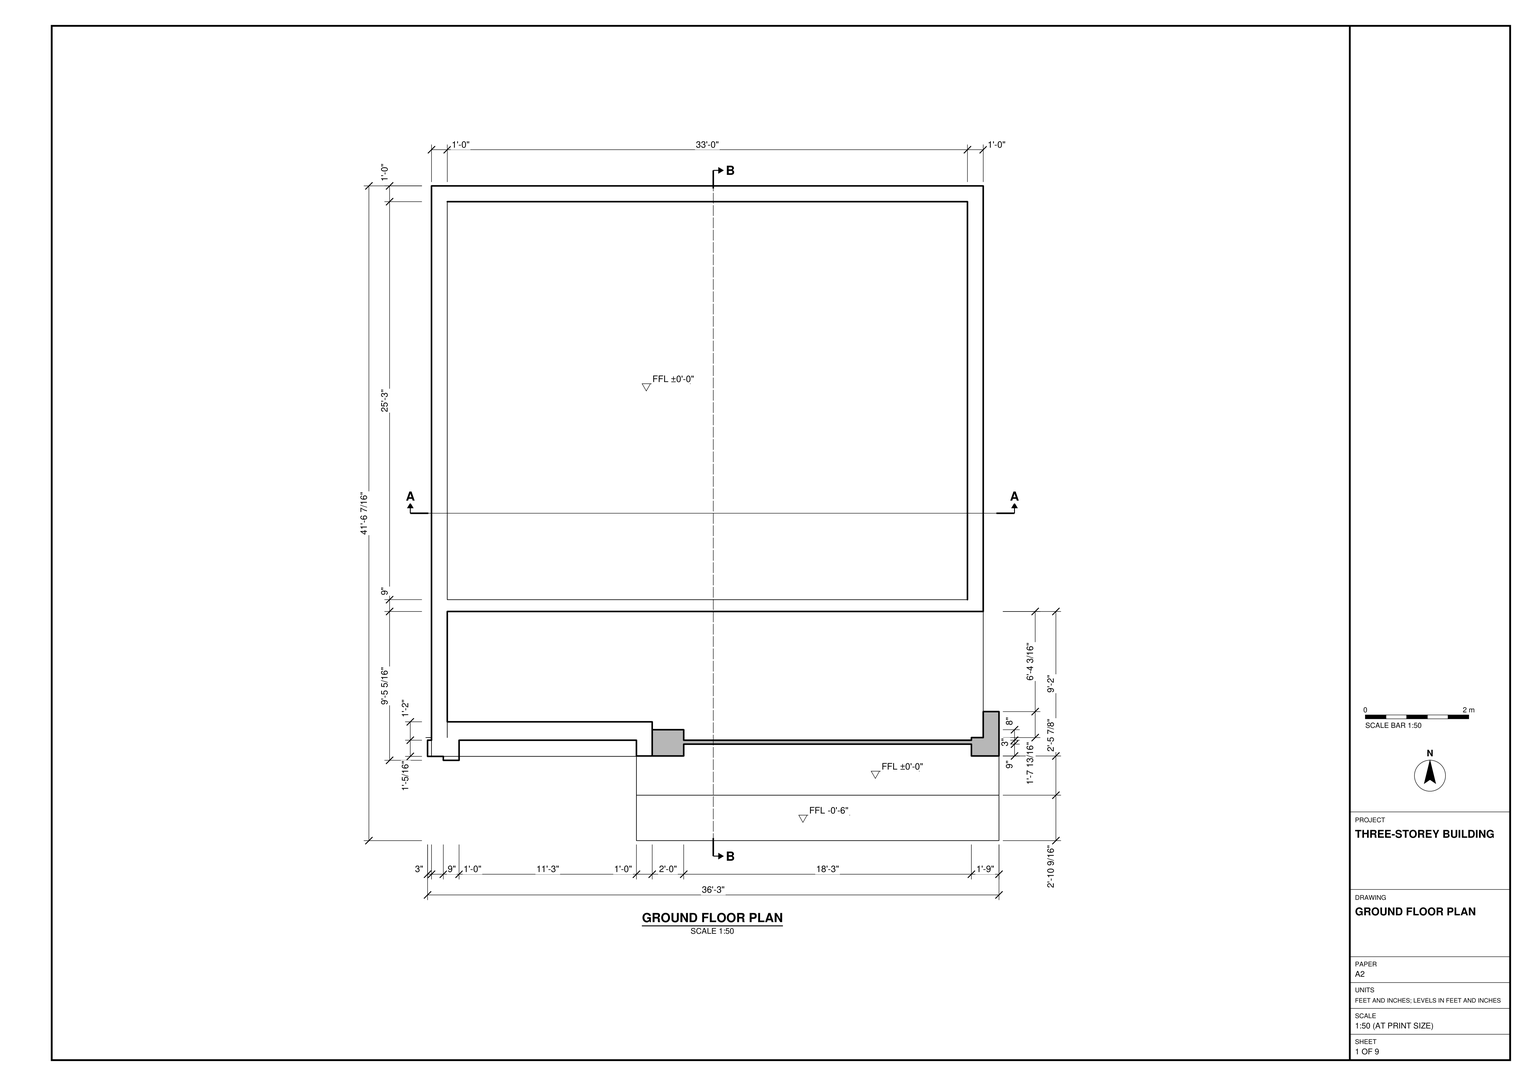
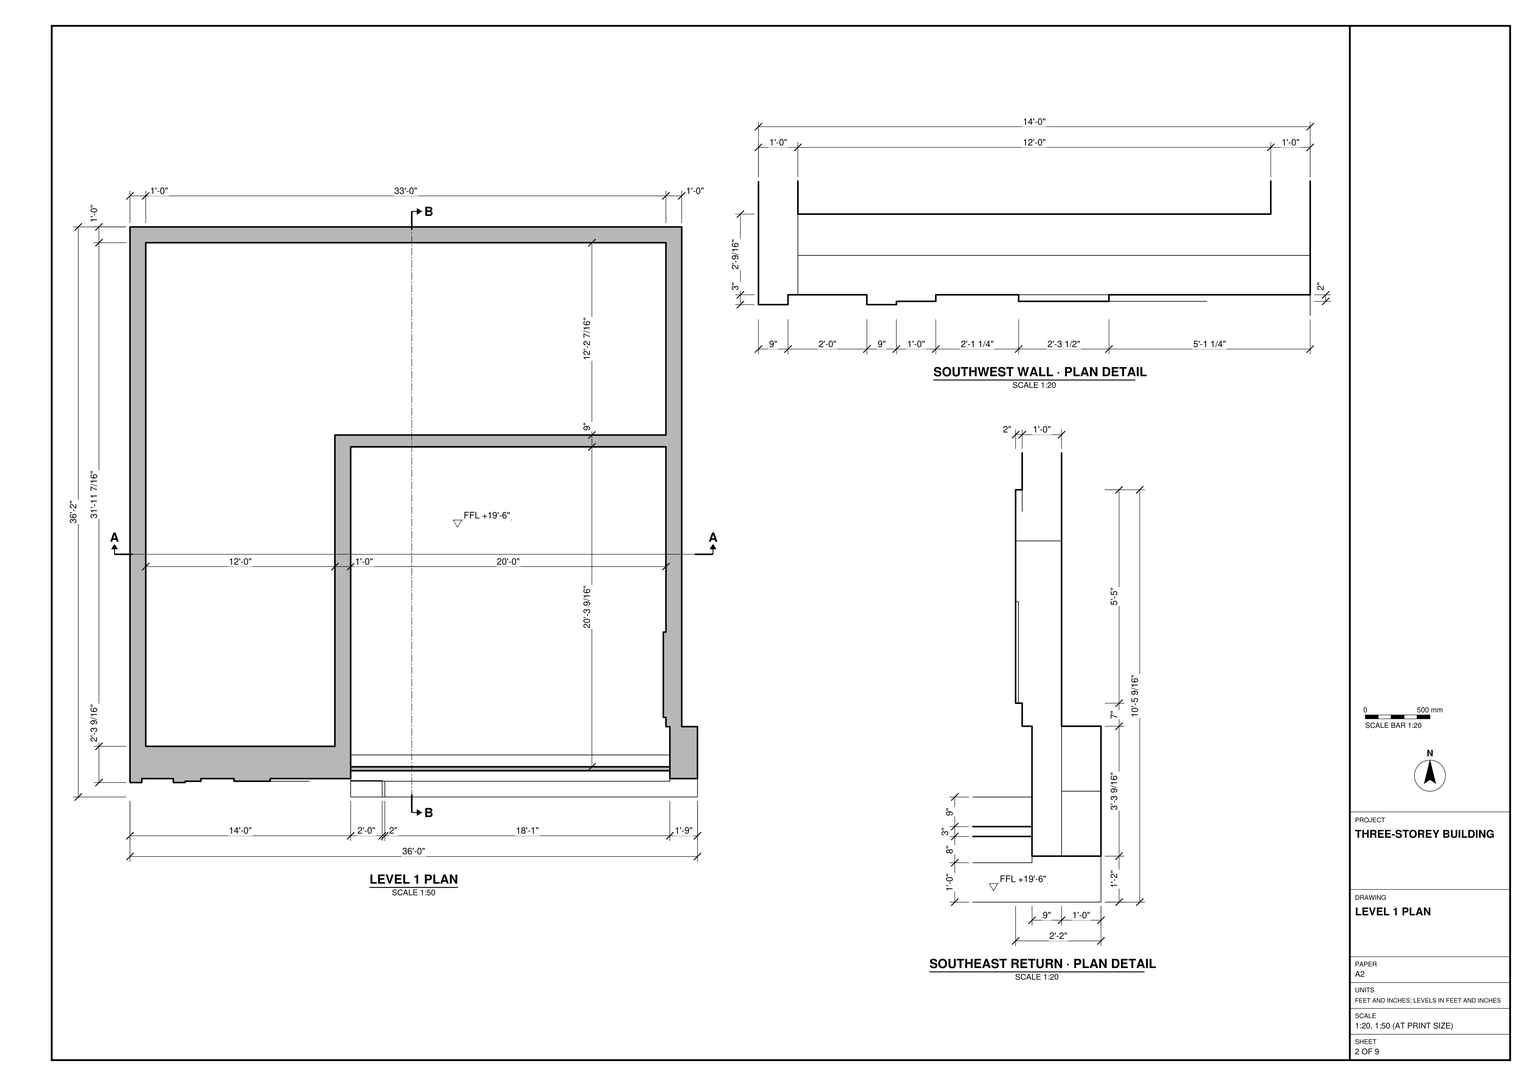
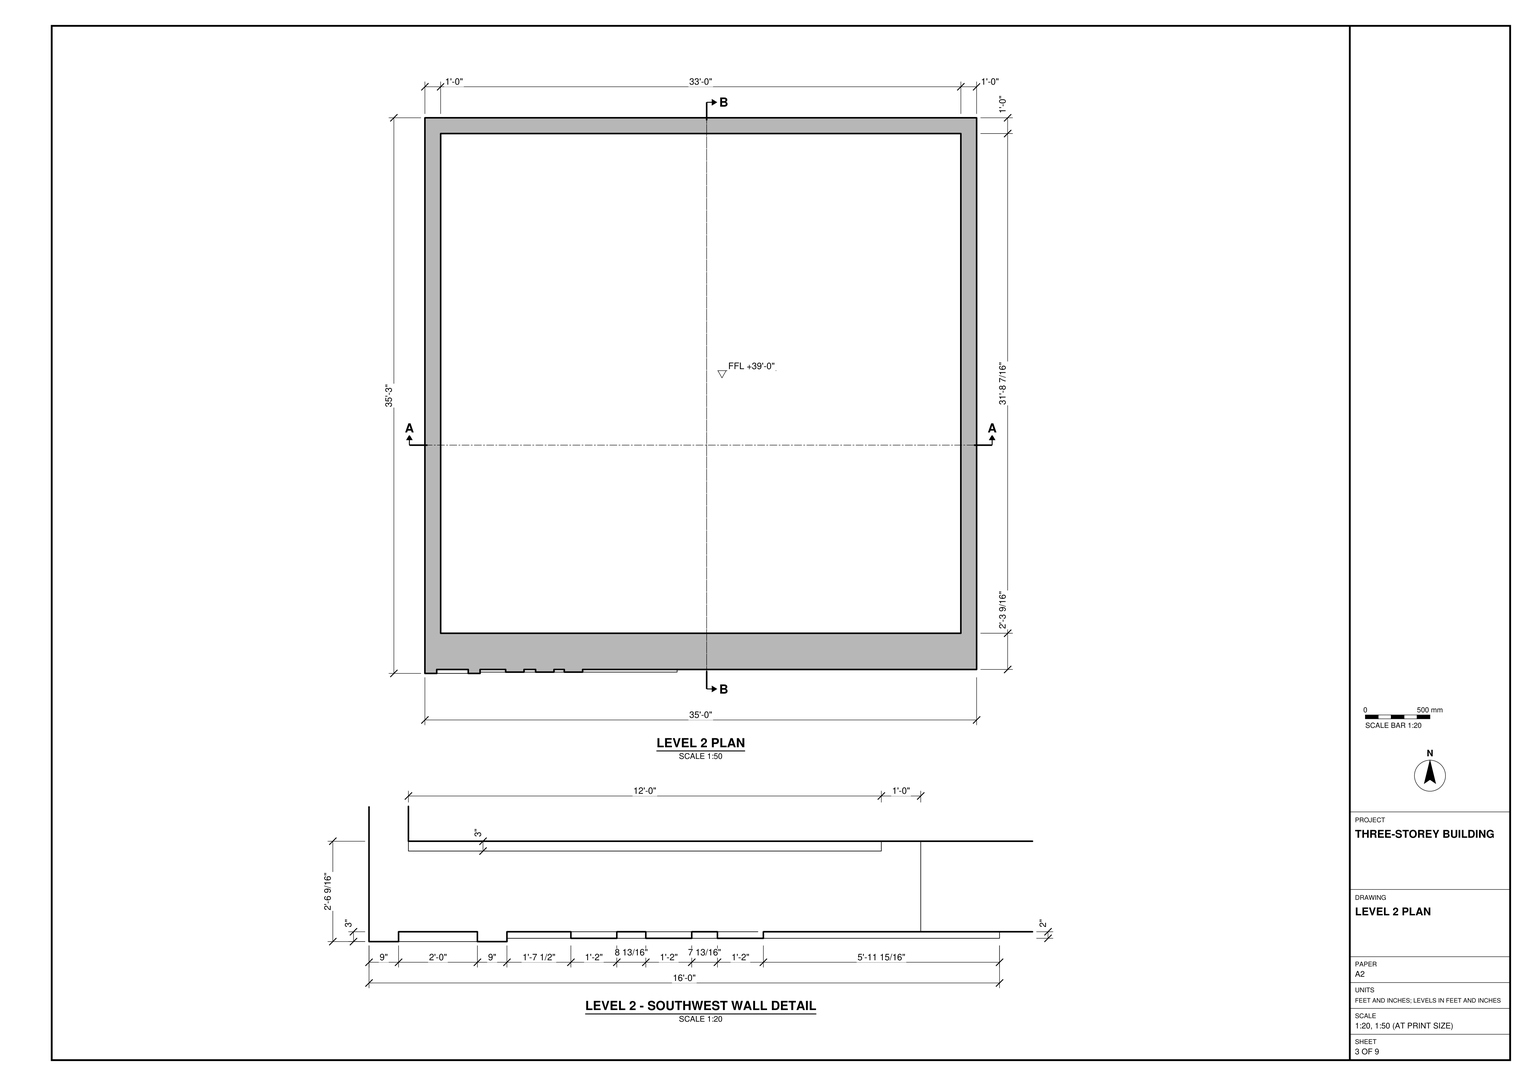
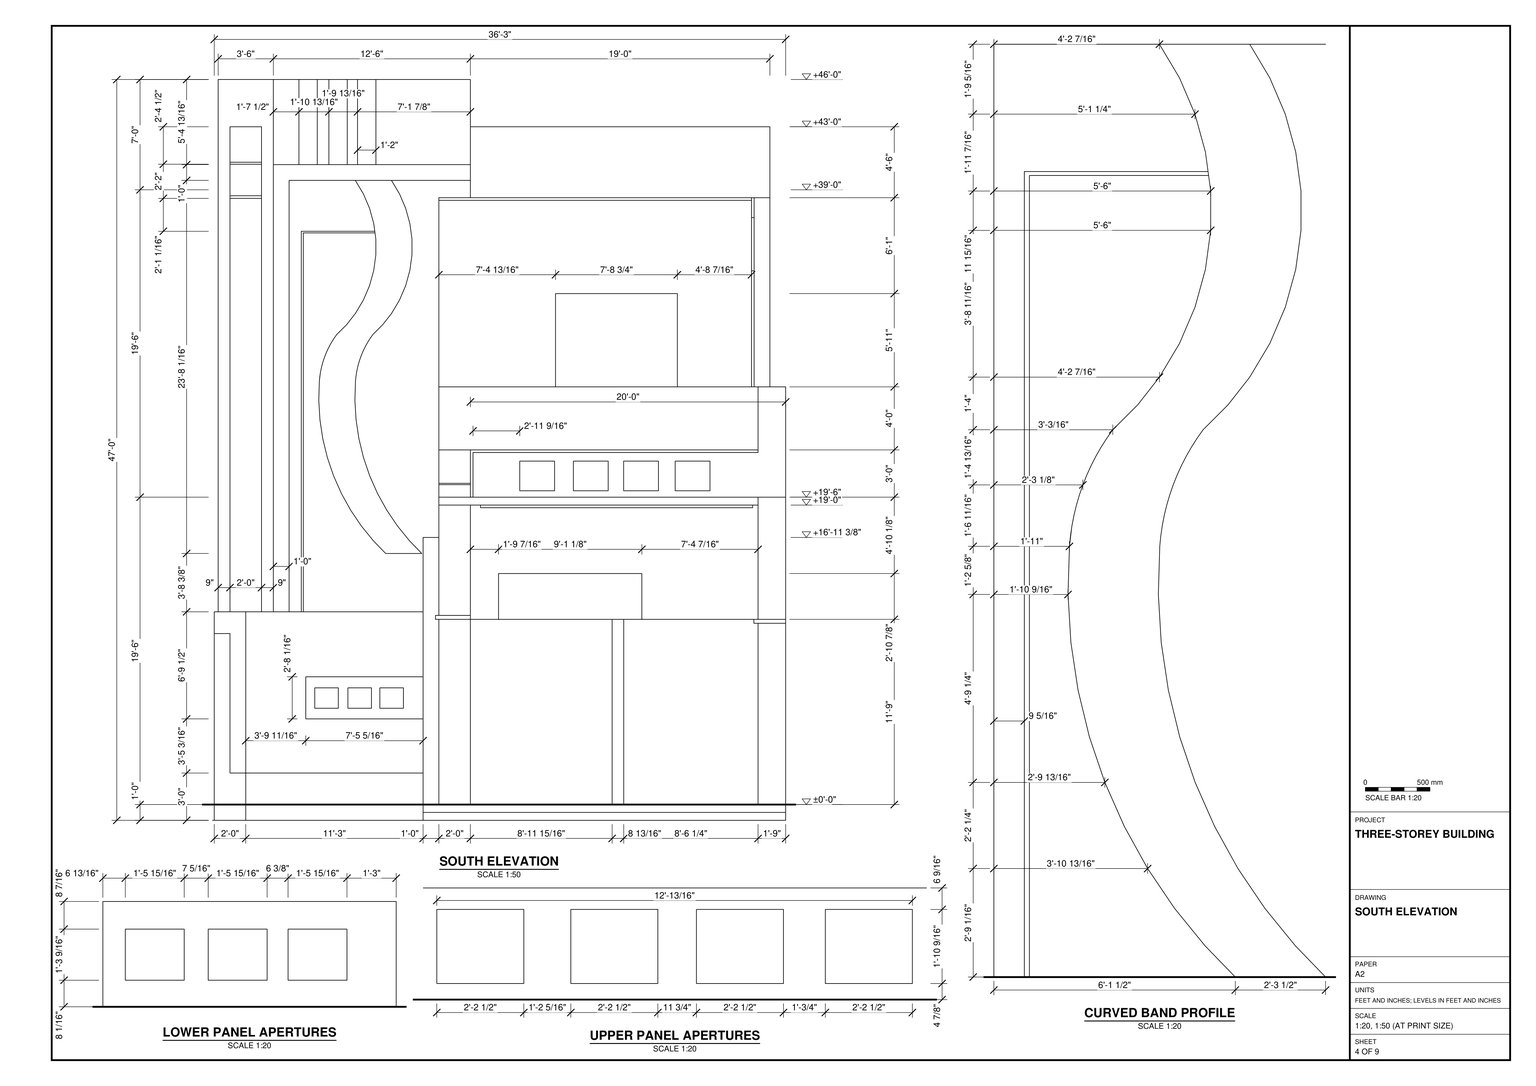
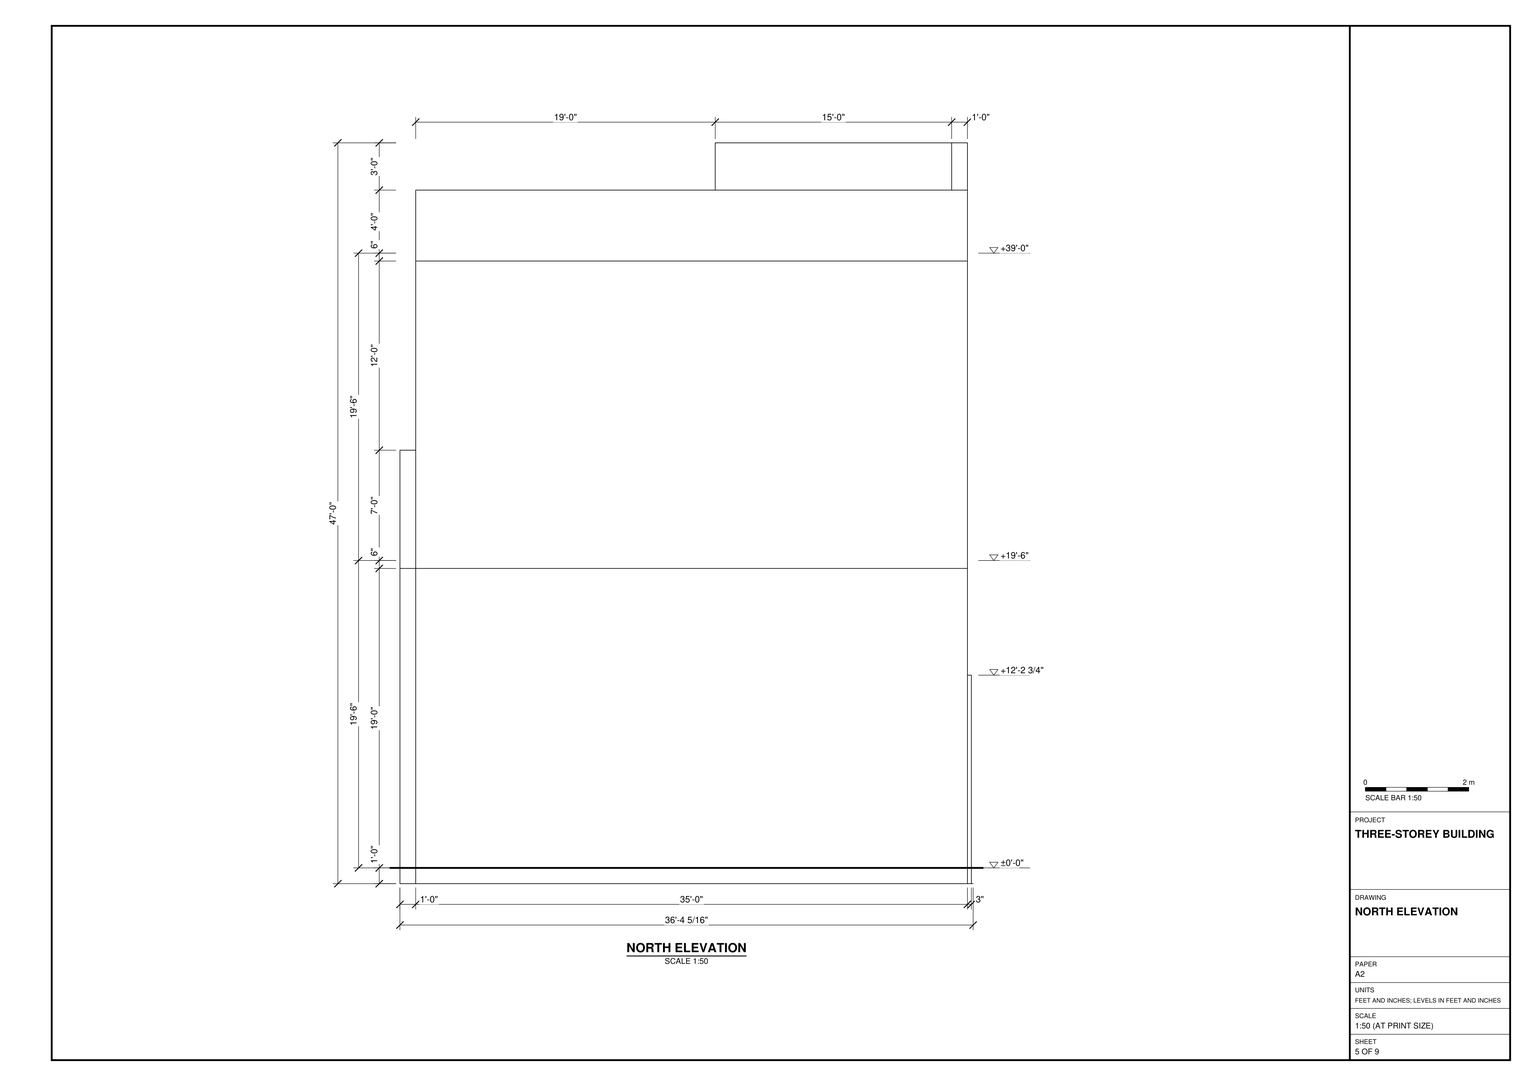
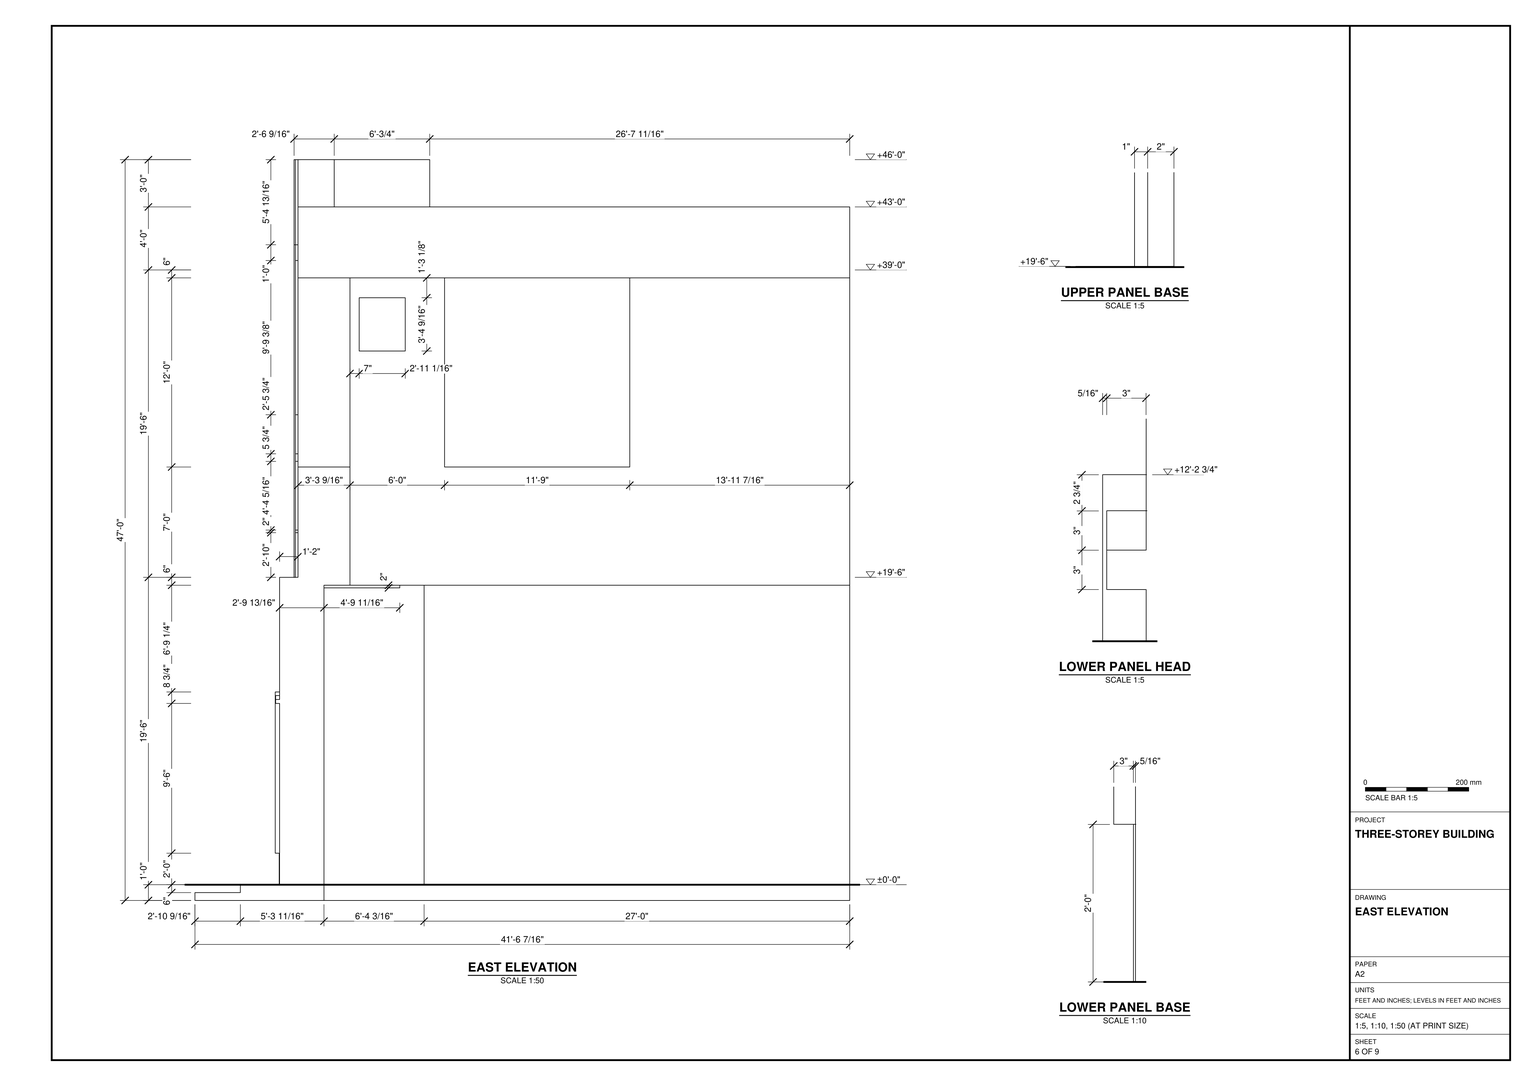
Build the three-storey shell in SketchUp from task_files/diagram_01.pdf. Work in feet and inches. Orient the south frontage along the x-axis. The overall model shall be 36'-3" wide, 41'-6 7/16" deep and 47'-0" high, including the projecting frontage and lower approach. Set the finished floor levels to ±0'-0", +19'-6" and +39'-0" relative to the ground floor.

Start with the rectangular ground-floor space. Use 1'-0" walls along its north, east and west sides and a 9" transverse wall separating it from the front zone. Model the stepped approach on the south side, including the lower strip in front of the eastern bay. At the middle level, use the Level 1 plan to locate the two walls that meet at the inset corner of the southeast bay. Follow the enlarged details for the offsets in the southwest wall face and the projecting southeast return. At the upper level, follow the rectangular perimeter and the thicker south edge. Use the sheets to resolve the openings, slab edges and roof profile rather than copying the same plan to every level.

Keep walls, slabs and roof elements in separate groups or components, do the same for each furniture or joinery piece shown, and use components for repeated parts. Any decor or loose items shown may be suitable library components. Save one SketchUp model as output_files/three_storey_building_with_its_stepped_south_frontage.skp.

# SketchUp Ruby script. Lengths in inches.
U = 1.inch
M = Sketchup.active_model
def pt(a) = Geom::Point3d.new(a.map { |v| v * U })
def face(e, loops, mat)
  f = e.add_face(loops[0].map { |a| pt(a) })
  loops[1..].each { |l| e.add_face(l.map { |a| pt(a) }).erase! }
  f.material = f.back_material = mat if mat
  f
end
# faces: each face lists its corners as indices into pts; further lists are holes
def faces(e, pts, list, mat = nil) = list.each { |f| face(e, (f[0].is_a?(Array) ? f : [f]).map { |l| l.map { |i| pts[i] } }, mat) }
# xy, xz, yz: faces in a plane at the given z, y or x. An outline is a flat list of corners, or four numbers for a rectangle; further outlines are holes
def ring(l) = l.size == 4 ? [[l[0], l[1]], [l[2], l[1]], [l[2], l[3]], [l[0], l[3]]] : l.each_slice(2).to_a
def flat(e, list, mat, &to3) = list.each { |f| face(e, (f[0].is_a?(Array) ? f : [f]).map { |l| ring(l).map { |u, v| to3.(u, v) } }, mat) }
def xy(e, z, list, mat = nil) = flat(e, list, mat) { |x, y| [x, y, z] }
def xz(e, y, list, mat = nil) = flat(e, list, mat) { |x, z| [x, y, z] }
def yz(e, x, list, mat = nil) = flat(e, list, mat) { |y, z| [x, y, z] }
def lines(e, pts, list) = list.each { |a, b| e.add_line(pt(pts[a]), pt(pts[b])) }
# prism: a flat outline (further loops are holes) pulled along v
def prism(e, loops, v, mat = nil)
  f = face(e, loops, mat); d = Geom::Vector3d.new(v.map { |x| x * U })
  f.pushpull(f.normal.samedirection?(d) ? d.length : -d.length)
end
def box(e, o, s, mat = nil) = prism(e, [[o, [o[0] + s[0], o[1], o[2]], [o[0] + s[0], o[1] + s[1], o[2]], [o[0], o[1] + s[1], o[2]]]], [0, 0, s[2]], mat)
def at(x, y, z, deg = 0) = Geom::Transformation.translation(pt([x, y, z])) * Geom::Transformation.rotation(ORIGIN, Z_AXIS, deg.degrees)
def axes(o, x, y, z) = Geom::Transformation.new([*x, 0, *y, 0, *z, 0, *pt(o).to_a, 1])
def part(name) = M.definitions.add(name)
# library, detail: a bought-in or finely detailed component or shape, given as its bounding box
def library(name, o, s) = part(name).tap { |d| box(d.entities, o, s) }
def detail(e, o, s) = box(e.add_group.entities, o, s)
def put(e, d, t, mat = nil) = e.add_instance(d, t).tap { |i| i.material = mat if mat }
def group(e, t, mat = nil) = e.add_group.tap { |g| g.transformation = t; g.material = mat if mat }.entities
root = M.entities
M.materials.add("[0005_LightPink]").color = [193, 138, 146]
M.materials.add("[0005_LightPink]1").color = [255, 182, 193]
M.materials.add("[0007_MistyRose]").color = [255, 228, 225]
M.materials.add("[0008_LavenderBlush]").color = [255, 240, 245]
M.materials.add("[0011_Seashell]").color = [255, 245, 238]
M.materials.add("[0012_Bisque]2").color = [255, 228, 196]
M.materials.add("[0013_LightCoral]").color = [255, 136, 136]
M.materials.add("[0013_LightCoral]1").color = [240, 128, 128]
M.materials.add("[0014_DarkSalmon]").color = [233, 150, 122]
M.materials.add("[0018_Brown]").color = [96, 24, 24]
M.materials.add("[0026_LightSalmon]").color = [255, 160, 122]
M.materials.add("[0111_SlateGray]").color = [112, 128, 144]
M.materials.add("[0119_RosyBrown]").color = [188, 143, 143]
M.materials.add("[0131_Silver]").color = [192, 192, 192]
M.materials.add("[0132_LightGray]").color = [169, 169, 169]
M.materials.add("[0136_Charcoal]").color = [35, 35, 35]
M.materials.add("[Brick Basket]").color = [230, 156, 152]
M.materials.add("[Brick Tumbled]").color = [135, 132, 132]
M.materials.add("[Carrera Marble]").color = [168, 168, 168]
M.materials.add("[Carrera Marble]1").color = [207, 207, 207]
M.materials.add("[Cladding Siding Tan]").color = [162, 126, 95]
M.materials.add("[Granite Dark Gray]").color = [69, 68, 68]
M.materials.add("[Stone Flagstone Ashlar]").color = [56, 37, 32]
M.materials.add("[Translucent Glass Gray]").color = [128, 128, 128]
M.materials["[Translucent Glass Gray]"].alpha = 0.5
M.materials.add("[Wood Cherry Original]").color = [152, 86, 42]
xy(root,0,[[159,0,159,76.4375,24,76.4375,24,64.125,3,64.125,3,498.4375,423,498.4375,423,98.221,435,98.221,435,0],[0,64.125,3,76.4375],[24,64.125,159,76.4375]])
xy(root,6,[[159,0,435,34.5625]],"[Granite Dark Gray]")
xy(root,12,[[171,64.4375,195,84.4375],[414,64.4375,435,78.4375],[195,73.4375,411,76.4375],[411,73.4375,414,76.4375],[423,78.4375,435,98.221],
  [15,183.4375,411,486.4375]])
xy(root,12,[[195,76.4375,414,76.4375,414,78.4375,423,78.4375,423,174.4375,15,174.4375,15,90.4375,171,90.4375,171,84.4375,195,84.4375]],"[Carrera Marble]")
xy(root,12,[[159,34.5625,435,34.5625,435,64.4375,414,64.4375,414,73.4375,195,73.4375,195,64.4375,159,64.4375]],"[Granite Dark Gray]")
xy(root,36,[[12,61.125,24,64.125]])
xy(root,36,[[24,64.125,159,76.4375]],"[Stone Flagstone Ashlar]")
xy(root,77.216,[[69.6875,70.4375,159,76.4375]],"[0111_SlateGray]")
xy(root,85.299,[[76.518,70.4375,94.455,72.4375],[101.768,70.4375,119.705,72.4375],[126.08,70.4375,144.018,72.4375]])
xy(root,100.862,[[76.518,70.4375,94.455,72.4375],[101.768,70.4375,119.705,72.4375],[126.08,70.4375,144.018,72.4375]])
xy(root,109.278,[[69.6875,70.4375,159,76.4375]],"[0111_SlateGray]")
xy(root,142.184,[[0,61.125,12,64.125]])
xy(root,150,[[410.8125,61.4375,410.8125,73.4375,414,73.4375,414,64.4375,435,64.4375,435,61.4375]])
xy(root,153,[[168.4375,61.4375,195,64.4375]])
xy(root,153,[[410.8125,61.4375,435,61.4375,435,64.4375,414,64.4375,414,76.4375,195,76.4375,195,73.4375,410.8125,73.4375]],"[0136_Charcoal]")
xy(root,156,[[168.4375,61.4375,195,61.4375,195,76.4375,171,76.4375,171,64.4375,168.4375,64.4375]],"[0013_LightCoral]")
xy(root,158.746,[[36,75.4375,45,76.4375]])
xy(root,158.746,[[0,61.125,24,61.125,24,76.4375,36,76.4375,36,78.4375,12,78.4375,12,75.4375,3,75.4375,3,76.4375,0,76.4375],[57,76.4375,159,78.4375]],"[0111_SlateGray]")
xy(root,203.132,[[130.514,76.4375,158.014,78.4375]],"[0026_LightSalmon]")
xy(root,215.357,[[171,78.4375,195,84.4375]])
xy(root,215.357,[[159,64.4375,171,78.4375]],"[0013_LightCoral]")
xy(root,238,[[237.548,105.396,235.982,105.433,234.479,105.874,233.141,106.689,232.06,107.822,231.309,109.197,230.94,110.719,230.976,112.285,231.417,113.788,232.232,115.125,233.366,116.207,234.74,116.958,236.262,117.327,237.828,117.29,239.331,116.849,240.669,116.034,241.75,114.901,242.501,113.527,242.87,112.004,242.834,110.439,242.393,108.936,241.578,107.598,240.444,106.517,239.07,105.766],[298.048,105.396,296.482,105.433,294.979,105.874,293.641,106.689,292.56,107.822,291.809,109.197,291.44,110.719,291.476,112.285,291.917,113.788,292.732,115.125,293.866,116.207,295.24,116.958,296.762,117.327,298.328,117.29,299.831,116.849,301.169,116.034,302.25,114.901,303.001,113.527,303.37,112.004,303.334,110.439,302.893,108.936,302.078,107.598,300.944,106.517,299.57,105.766],[341.735,105.396,340.169,105.433,338.666,105.874,337.329,106.689,336.248,107.822,335.497,109.197,335.127,110.719,335.164,112.285,335.605,113.788,336.42,115.125,337.553,116.207,338.928,116.958,340.45,117.327,342.016,117.29,343.519,116.849,344.856,116.034,345.9375,114.901,346.688,113.527,347.058,112.004,347.021,110.439,346.58,108.936,345.765,107.598,344.632,106.517,343.257,105.766],[386.048,105.396,384.482,105.433,382.979,105.874,381.641,106.689,380.56,107.822,379.809,109.197,379.44,110.719,379.476,112.285,379.917,113.788,380.732,115.125,381.866,116.207,383.24,116.958,384.762,117.327,386.328,117.29,387.831,116.849,389.169,116.034,390.25,114.901,391.001,113.527,391.37,112.004,391.334,110.439,390.893,108.936,390.078,107.598,388.944,106.517,387.57,105.766]])
xy(root,238,[[[202.693,81.739,409.88,155.927],[298.048,105.396,299.57,105.766,300.944,106.517,302.078,107.598,302.893,108.936,303.334,110.439,303.37,112.004,303.001,113.527,302.25,114.901,301.169,116.034,299.831,116.849,298.328,117.29,296.762,117.327,295.24,116.958,293.866,116.207,292.732,115.125,291.917,113.788,291.476,112.285,291.44,110.719,291.809,109.197,292.56,107.822,293.641,106.689,294.979,105.874,296.482,105.433],[386.048,105.396,387.57,105.766,388.944,106.517,390.078,107.598,390.893,108.936,391.334,110.439,391.37,112.004,391.001,113.527,390.25,114.901,389.169,116.034,387.831,116.849,386.328,117.29,384.762,117.327,383.24,116.958,381.866,116.207,380.732,115.125,379.917,113.788,379.476,112.285,379.44,110.719,379.809,109.197,380.56,107.822,381.641,106.689,382.979,105.874,384.482,105.433],[341.735,105.396,343.257,105.766,344.632,106.517,345.765,107.598,346.58,108.936,347.021,110.439,347.058,112.004,346.688,113.527,345.9375,114.901,344.856,116.034,343.519,116.849,342.016,117.29,340.45,117.327,338.928,116.958,337.553,116.207,336.42,115.125,335.605,113.788,335.164,112.285,335.127,110.719,335.497,109.197,336.248,107.822,337.329,106.689,338.666,105.874,340.169,105.433],[237.548,105.396,239.07,105.766,240.444,106.517,241.578,107.598,242.393,108.936,242.834,110.439,242.87,112.004,242.501,113.527,241.75,114.901,240.669,116.034,239.331,116.849,237.828,117.29,236.262,117.327,234.74,116.958,233.366,116.207,232.232,115.125,231.417,113.788,230.976,112.285,230.94,110.719,231.309,109.197,232.06,107.822,233.141,106.689,234.479,105.874,235.982,105.433]]],"[Wood Cherry Original]")
xy(root,240,[[321.222,67.739,319.656,67.776,318.153,68.217,316.816,69.032,315.734,70.165,314.983,71.54,314.614,73.062,314.651,74.628,315.092,76.131,315.906,77.468,317.04,78.549,318.414,79.3,319.936,79.67,321.502,79.633,323.005,79.192,324.343,78.377,325.424,77.244,326.175,75.869,326.545,74.347,326.508,72.782,326.067,71.279,325.252,69.941,324.119,68.86,322.744,68.109],[423,98.221,435,118.005]])
xy(root,240,[[[171,64.4375,171,76.4375,195,76.4375,195,78.4375,171,78.4375,171,90.4375,15,90.4375,15,174.4375,423,174.4375,423,78.4375,414,78.4375,414,64.4375],[202.693,81.739,409.88,155.927],[321.222,67.739,322.744,68.109,324.119,68.86,325.252,69.941,326.067,71.279,326.508,72.782,326.545,74.347,326.175,75.869,325.424,77.244,324.343,78.377,323.005,79.192,321.502,79.633,319.936,79.67,318.414,79.3,317.04,78.549,315.906,77.468,315.092,76.131,314.651,74.628,314.614,73.062,314.983,71.54,315.734,70.165,316.816,69.032,318.153,68.217,319.656,67.776]]],"[0007_MistyRose]")
xy(root,246,[[195,76.4375,197,78.4375],[171,77,195,78.4375],[15,103.005,159,103.005,159,340.005,411,340.005,411,486.4375,15,486.4375]])
xy(root,246,[[171,64.4375,195,77],[195,64.4375,197,76.4375],[197,64.4375,435,78.4375]],"[0111_SlateGray]")
xy(root,246,[[171,96.4375,414,96.4375,414,118.005,411,118.005,411,125.019,409,125.019,409,190.005,411,190.005,411,331.005,171,331.005]],"[Carrera Marble]")
xy(root,250.897,[[232.592,78.4375,259.092,81.4375],[273.405,78.4375,299.905,81.4375],[311.655,78.4375,338.155,81.4375],[350.905,78.4375,377.405,81.4375]],"[0111_SlateGray]")
xy(root,255.554,[[171,76.4375,195,77]])
xy(root,256.554,[[171,76.4375,195,77]])
xy(root,273.46,[[232.592,78.4375,259.092,81.4375],[273.405,78.4375,299.905,81.4375],[311.655,78.4375,338.155,81.4375],[350.905,78.4375,377.405,81.4375]])
xy(root,280,[[197,76.4375,414,78.4375]],"[0111_SlateGray]")
xy(root,282,[[171,84.4375,414,96.4375]])
xy(root,282,[[195,76.4375,414,76.4375,414,84.4375,171,84.4375,171,77,195,77]],"[0111_SlateGray]")
xy(root,330,[[411,190.005,423,331.005]],"[0005_LightPink]1")
xy(root,330,[[414,78.4375,435,118.005],[171,84.4375,414,87.4375]],"[0013_LightCoral]")
xy(root,418.301,[[409,125.019,423,160.081]],"[0005_LightPink]1")
xy(root,472,[[171,185.005,409,190.005]],"[Wood Cherry Original]")
xy(root,473.496,[[12,75.4375,36,78.4375]])
xy(root,474,[[218.054,111.37,216.501,111.574,215.054,112.173,213.812,113.127,212.858,114.37,212.259,115.817,212.054,117.37,212.259,118.923,212.858,120.37,213.812,121.612,215.054,122.566,216.501,123.165,218.054,123.37,219.607,123.165,221.054,122.566,222.297,121.612,223.25,120.37,223.85,118.923,224.054,117.37,223.85,115.817,223.25,114.37,222.297,113.127,221.054,112.173,219.607,111.574],[319.992,111.37,318.439,111.574,316.992,112.173,315.749,113.127,314.796,114.37,314.196,115.817,313.992,117.37,314.196,118.923,314.796,120.37,315.749,121.612,316.992,122.566,318.439,123.165,319.992,123.37,321.545,123.165,322.992,122.566,324.234,121.612,325.188,120.37,325.787,118.923,325.992,117.37,325.787,115.817,325.188,114.37,324.234,113.127,322.992,112.173,321.545,111.574],[219.3,215.462,217.747,215.666,216.3,216.266,215.058,217.219,214.104,218.462,213.505,219.909,213.3,221.462,213.505,223.015,214.104,224.462,215.058,225.705,216.3,226.658,217.747,227.258,219.3,227.462,220.853,227.258,222.3,226.658,223.543,225.705,224.497,224.462,225.096,223.015,225.3,221.462,225.096,219.909,224.497,218.462,223.543,217.219,222.3,216.266,220.853,215.666],[290.738,215.462,289.185,215.666,287.738,216.266,286.495,217.219,285.542,218.462,284.942,219.909,284.738,221.462,284.942,223.015,285.542,224.462,286.495,225.705,287.738,226.658,289.185,227.258,290.738,227.462,292.291,227.258,293.738,226.658,294.981,225.705,295.934,224.462,296.533,223.015,296.738,221.462,296.533,219.909,295.934,218.462,294.981,217.219,293.738,216.266,292.291,215.666],[372.738,215.462,371.185,215.666,369.738,216.266,368.495,217.219,367.542,218.462,366.942,219.909,366.738,221.462,366.942,223.015,367.542,224.462,368.495,225.705,369.738,226.658,371.185,227.258,372.738,227.462,374.291,227.258,375.738,226.658,376.981,225.705,377.934,224.462,378.533,223.015,378.738,221.462,378.533,219.909,377.934,218.462,376.981,217.219,375.738,216.266,374.291,215.666]])
xy(root,474,[[[171,78.4375,171,185.005,409,185.005,409,160.081,411,160.081,411,118.005,423,118.005,423,78.4375],[218.054,111.37,219.607,111.574,221.054,112.173,222.297,113.127,223.25,114.37,223.85,115.817,224.054,117.37,223.85,118.923,223.25,120.37,222.297,121.612,221.054,122.566,219.607,123.165,218.054,123.37,216.501,123.165,215.054,122.566,213.812,121.612,212.858,120.37,212.259,118.923,212.054,117.37,212.259,115.817,212.858,114.37,213.812,113.127,215.054,112.173,216.501,111.574],[319.992,111.37,321.545,111.574,322.992,112.173,324.234,113.127,325.188,114.37,325.787,115.817,325.992,117.37,325.787,118.923,325.188,120.37,324.234,121.612,322.992,122.566,321.545,123.165,319.992,123.37,318.439,123.165,316.992,122.566,315.749,121.612,314.796,120.37,314.196,118.923,313.992,117.37,314.196,115.817,314.796,114.37,315.749,113.127,316.992,112.173,318.439,111.574]],[[171,190.005,423,331.005],[290.738,215.462,292.291,215.666,293.738,216.266,294.981,217.219,295.934,218.462,296.533,219.909,296.738,221.462,296.533,223.015,295.934,224.462,294.981,225.705,293.738,226.658,292.291,227.258,290.738,227.462,289.185,227.258,287.738,226.658,286.495,225.705,285.542,224.462,284.942,223.015,284.738,221.462,284.942,219.909,285.542,218.462,286.495,217.219,287.738,216.266,289.185,215.666],[372.738,215.462,374.291,215.666,375.738,216.266,376.981,217.219,377.934,218.462,378.533,219.909,378.738,221.462,378.533,223.015,377.934,224.462,376.981,225.705,375.738,226.658,374.291,227.258,372.738,227.462,371.185,227.258,369.738,226.658,368.495,225.705,367.542,224.462,366.942,223.015,366.738,221.462,366.942,219.909,367.542,218.462,368.495,217.219,369.738,216.266,371.185,215.666],[219.3,215.462,220.853,215.666,222.3,216.266,223.543,217.219,224.497,218.462,225.096,219.909,225.3,221.462,225.096,223.015,224.497,224.462,223.543,225.705,222.3,226.658,220.853,227.258,219.3,227.462,217.747,227.258,216.3,226.658,215.058,225.705,214.104,224.462,213.505,223.015,213.3,221.462,213.505,219.909,214.104,218.462,215.058,217.219,216.3,216.266,217.747,215.666]]],"[Wood Cherry Original]")
xy(root,475.496,[[12,75.4375,36,78.4375]])
xy(root,480,[[15,106.005,411,486.4375]])
xy(root,487.191,[[57,76.4375,107.413,78.4375],[134.913,76.4375,195,78.4375]])
xy(root,499.191,[[45,76.4375,64.474,78.4375],[78.457,76.4375,87.286,78.4375],[101.27,76.4375,109.099,78.4375],[123.082,76.4375,195,78.4375]])
xy(root,499.496,[[12,75.4375,36,78.4375]])
xy(root,500.996,[[12,75.4375,36,78.4375]])
xy(root,528,[[12,75.4375,36,78.4375],[195,78.4375,423,78.4375,423,498.4375,3,498.4375,3,178.725,15,178.725,15,486.4375,411,486.4375,411,106.005,195,106.005]])
xy(root,564,[[3,75.4375,45,75.4375,45,78.4375,64.474,78.4375,64.474,76.4375,78.457,76.4375,78.457,78.4375,87.286,78.4375,87.286,76.4375,101.27,76.4375,101.27,78.4375,109.099,78.4375,109.099,76.4375,123.082,76.4375,123.082,78.4375,195,78.4375,195,106.005,15,106.005,15,178.725,3,178.725]])
xz(root,0,[[159,0,435,6]],"[Granite Dark Gray]")
xz(root,34.5625,[[159,6,435,12]],"[Granite Dark Gray]")
xz(root,61.125,[[12,36,24,36,24,158.746,0,158.746,0,142.184,12,142.184]],"[0111_SlateGray]")
xz(root,61.4375,[[168.4375,153,195,156]])
xz(root,61.4375,[[410.8125,150,435,153]],"[0013_LightCoral]")
xz(root,64.125,[[0,0,24,0,24,36,12,36,12,142.184,0,142.184],[24,0,159,36]],"[Stone Flagstone Ashlar]")
xz(root,64.4375,[[168.4375,153,171,156]])
xz(root,64.4375,[[159,12,171,12,171,153,168.4375,153,168.4375,156,171,156,171,215.357,159,215.357],[171,12,195,153],[414,12,435,150],[414,153,435,246]],"[0013_LightCoral]")
xz(root,64.4375,[[171,240,414,246]],"[0111_SlateGray]")
xz(root,70.4375,[[[69.6875,77.216,159,109.278],[76.518,85.299,94.455,100.862],[101.768,85.299,119.705,100.862],[126.08,85.299,144.018,100.862]]],"[0111_SlateGray]")
xz(root,72.4375,[[76.518,85.299,94.455,100.862],[101.768,85.299,119.705,100.862],[126.08,85.299,144.018,100.862]])
xz(root,73.4375,[[302.906,12,311.725,153]],"[0136_Charcoal]")
xz(root,73.4375,[[195,12,302.906,153],[311.725,12,414,12,414,150,410.8125,150,410.8125,153,311.725,153]],"[Cladding Siding Tan]")
xz(root,75.4375,[[12,473.496,36,475.496],[12,499.496,36,500.996]],"[0012_Bisque]2")
xz(root,75.4375,[[3,158.746,12,158.746,12,528,36,528,36,158.746,45,158.746,45,564,3,564]],"[Brick Basket]")
xz(root,76.4375,[[0,0,3,158.746],[24,0,159,36]])
xz(root,76.4375,[[45,158.746,57,158.746,57,487.191,195,487.191,195,499.191,45,499.191]],"[0005_LightPink]")
xz(root,76.4375,[[64.474,499.191,78.457,564],[87.286,499.191,101.27,564],[109.099,499.191,123.082,564]],"[0011_Seashell]")
xz(root,76.4375,[[171,156,195,240]],"[0013_LightCoral]")
xz(root,76.4375,[[130.514,203.132,158.014,203.132,148.792,212.666,139.533,224.026,131.322,236.166,124.225,248.988,118.298,262.391,113.588,276.269,110.132,290.51,107.958,305.004,107.084,319.633,107.515,334.281,107.826,337.465,108.202,340.047,108.287,340.631,108.895,343.771,109.651,346.879,110.551,349.949,111.595,352.973,112.779,355.944,114.102,358.857,115.559,361.704,117.149,364.48,118.868,367.178,120.711,369.792,128.295,377.376,134.913,385.816,141.044,396.099,145.741,407.111,148.921,418.653,150.525,430.517,150.525,442.489,148.921,454.353,145.741,465.895,141.044,476.907,134.913,487.191,107.413,487.191,113.544,476.907,118.241,465.895,121.421,454.353,123.025,442.489,123.025,430.517,121.421,418.653,118.241,407.111,113.544,396.099,107.413,385.816,100.795,377.376,93.211,369.792,91.368,367.178,89.649,364.48,88.059,361.704,86.602,358.857,85.279,355.944,84.095,352.973,83.051,349.949,82.151,346.879,81.395,343.771,80.787,340.631,80.702,340.047,80.015,334.281,79.584,319.633,80.458,305.004,82.632,290.51,86.088,276.269,90.798,262.391,96.725,248.988,103.822,236.166,112.033,224.026,121.292,212.666]],"[0026_LightSalmon]")
xz(root,76.4375,[[195,246,197,246,197,280,414,280,414,282,195,282],[171,255.554,195,256.554]],"[0111_SlateGray]")
xz(root,76.4375,[[24,36,159,36,159,77.216,69.6875,77.216,69.6875,109.278,159,109.278,159,158.746,24,158.746]],"[0132_LightGray]")
xz(root,76.4375,[[195,12,414,153]],"[Cladding Siding Tan]")
xz(root,77,[[171,246,195,255.554],[171,256.554,195,282]],"[0111_SlateGray]")
xz(root,78.4375,[[414,12,423,240],[66.285,158.746,67.823,158.746,67.823,447.223,122.385,447.223,122.223,448.421,66.285,448.421],[171,215.357,195,240],[80.015,334.281,80.702,340.047,80.326,337.465]])
xz(root,78.4375,[[57,158.746,66.285,158.746,66.285,448.421,122.223,448.421,121.421,454.353,118.241,465.895,113.544,476.907,107.413,487.191,57,487.191]],"[0005_LightPink]")
xz(root,78.4375,[[[197,246,435,246,435,330,414,330,414,280,197,280],[350.905,250.897,377.405,273.46],[311.655,250.897,338.155,273.46],[273.405,250.897,299.905,273.46],[232.592,250.897,259.092,273.46]]],"[0013_LightCoral]")
xz(root,78.4375,[[67.823,158.746,159,158.746,159,215.357,171,215.357,171,474,195,474,195,487.191,134.913,487.191,141.044,476.907,145.741,465.895,148.921,454.353,150.525,442.489,150.525,430.517,148.921,418.653,145.741,407.111,141.044,396.099,134.913,385.816,128.295,377.376,120.711,369.792,118.868,367.178,117.149,364.48,115.559,361.704,114.102,358.857,112.779,355.944,111.595,352.973,110.551,349.949,109.651,346.879,108.895,343.771,108.287,340.631,108.202,340.047,107.826,337.465,107.515,334.281,107.084,319.633,107.958,305.004,110.132,290.51,113.588,276.269,118.298,262.391,124.225,248.988,131.322,236.166,139.533,224.026,148.792,212.666,158.014,203.132,130.514,203.132,121.292,212.666,112.033,224.026,103.822,236.166,96.725,248.988,90.798,262.391,86.088,276.269,82.632,290.51,80.458,305.004,79.584,319.633,80.015,334.281,80.326,337.465,80.702,340.047,80.787,340.631,81.395,343.771,82.151,346.879,83.051,349.949,84.095,352.973,85.279,355.944,86.602,358.857,88.059,361.704,89.649,364.48,91.368,367.178,93.211,369.792,100.795,377.376,107.413,385.816,113.544,396.099,118.241,407.111,121.421,418.653,123.025,430.517,123.025,442.489,122.385,447.223,67.823,447.223]],"[0119_RosyBrown]")
xz(root,78.4375,[[45,499.191,64.474,564],[78.457,499.191,87.286,564],[101.27,499.191,109.099,564],[123.082,499.191,195,564]],"[Brick Basket]")
xz(root,78.4375,[[195,474,423,528]],"[Brick Tumbled]")
xz(root,78.4375,[[12,158.746,36,473.496],[12,475.496,36,499.496],[12,500.996,36,528]],"[Translucent Glass Gray]")
xz(root,81.4375,[[232.592,250.897,259.092,273.46],[273.405,250.897,299.905,273.46],[311.655,250.897,338.155,273.46],[350.905,250.897,377.405,273.46]],"[0111_SlateGray]")
xz(root,81.739,[[202.693,238,409.88,240]],"[Wood Cherry Original]")
xz(root,84.4375,[[171,12,195,215.357]],"[0007_MistyRose]")
xz(root,84.4375,[[171,282,414,330]],"[0013_LightCoral]")
xz(root,87.4375,[[171,282,414,330]])
xz(root,90.4375,[[15,12,171,240]],"[0007_MistyRose]")
xz(root,96.4375,[[171,246,414,282]])
xz(root,98.221,[[423,0,435,12]])
xz(root,98.221,[[423,12,435,240]],"[0013_LightCoral]1")
xz(root,103.005,[[15,246,159,474]])
xz(root,106.005,[[15,480,195,564],[195,480,411,528]])
xz(root,118.005,[[423,240,435,330]],"[0013_LightCoral]1")
xz(root,118.005,[[411,246,414,246,414,330,423,330,423,474,411,474]],"[0111_SlateGray]")
xz(root,125.019,[[411,418.301,423,458.863]])
xz(root,125.019,[[409,246,411,418.301]],"[0005_LightPink]1")
xz(root,155.927,[[202.693,238,409.88,240]])
xz(root,160.081,[[409,458.857,411,458.863],[409,458.863,411,474]])
xz(root,160.081,[[409,418.301,423,458.857]],"[0005_LightPink]1")
xz(root,174.4375,[[221.441,89.955,224.754,104.205]],"[0007_MistyRose]")
xz(root,174.4375,[[[216.433,12,325.533,187.875],[221.441,89.955,224.754,104.205]]],"[0018_Brown]")
xz(root,174.4375,[[15,12,216.433,12,216.433,187.875,325.533,187.875,325.533,12,423,12,423,240,15,240]],"[Carrera Marble]1")
xz(root,178.725,[[3,528,15,564]])
xz(root,185.005,[[171,472,409,474]],"[Wood Cherry Original]")
xz(root,190.005,[[409,246,411,330],[409,330,409,472,411,472,411,474,423,474,423,330],[171,472,411,474]])
xz(root,331.005,[[411,330,423,474]],"[0005_LightPink]1")
xz(root,331.005,[[269.301,317.864,270.073,317.993,270.786,318.317,271.391,318.814,271.847,319.451,272.122,320.185,272.198,320.964,272.069,321.737,271.745,322.45,271.248,323.054,270.611,323.51,269.878,323.785,269.098,323.861,268.326,323.733,267.613,323.409,267.008,322.911,266.552,322.274,266.277,321.541,266.201,320.761,266.329,319.989,266.653,319.276,267.151,318.671,267.788,318.215,268.521,317.94]],"[0008_LavenderBlush]")
xz(root,331.005,[[[259.809,246,352.559,401],[269.301,317.864,268.521,317.94,267.788,318.215,267.151,318.671,266.653,319.276,266.329,319.989,266.201,320.761,266.277,321.541,266.552,322.274,267.008,322.911,267.613,323.409,268.326,323.733,269.098,323.861,269.878,323.785,270.611,323.51,271.248,323.054,271.745,322.45,272.069,321.737,272.198,320.964,272.122,320.185,271.847,319.451,271.391,318.814,270.786,318.317,270.073,317.993]]],"[0018_Brown]")
xz(root,331.005,[[171,246,259.809,246,259.809,401,352.559,401,352.559,246,411,246,411,474,171,474]],"[Carrera Marble]1")
xz(root,340.005,[[159,246,411,474]])
xz(root,486.4375,[[15,12,411,240],[15,246,411,474],[15,480,411,528]])
xz(root,498.4375,[[3,0,423,240],[3,240,423,474],[3,474,423,528]])
yz(root,0,[[64.125,0,64.125,142.184,61.125,142.184,61.125,158.746,76.4375,158.746,76.4375,0]])
yz(root,3,[[76.4375,0,76.4375,158.746,75.4375,158.746,75.4375,564,178.725,564,178.725,528,498.4375,528,498.4375,0]],"[0007_MistyRose]")
yz(root,12,[[61.125,36,64.125,142.184]])
yz(root,12,[[75.4375,158.746,78.4375,473.496],[75.4375,475.496,78.4375,499.496],[75.4375,500.996,78.4375,528]],"[0131_Silver]")
yz(root,15,[[103.005,246,486.4375,474],[106.005,480,178.725,564],[178.725,480,486.4375,528]])
yz(root,15,[[90.4375,12,174.4375,240]],"[0007_MistyRose]")
yz(root,24,[[64.125,0,76.4375,36]])
yz(root,24,[[61.125,36,76.4375,158.746]],"[0111_SlateGray]")
yz(root,36,[[75.4375,158.746,78.4375,473.496]])
yz(root,36,[[75.4375,475.496,78.4375,499.496],[75.4375,500.996,78.4375,528]],"[0131_Silver]")
yz(root,45,[[75.4375,158.746,76.4375,499.191],[75.4375,499.191,78.4375,564]])
yz(root,57,[[76.4375,158.746,78.4375,487.191]])
yz(root,64.474,[[76.4375,499.191,78.4375,564]])
yz(root,69.6875,[[70.4375,77.216,76.4375,109.278]],"[0111_SlateGray]")
yz(root,76.518,[[70.4375,85.299,72.4375,100.862]])
yz(root,78.457,[[76.4375,499.191,78.4375,564]])
yz(root,87.286,[[76.4375,499.191,78.4375,564]])
yz(root,94.455,[[70.4375,85.299,72.4375,100.862]])
yz(root,101.27,[[76.4375,499.191,78.4375,564]])
yz(root,101.768,[[70.4375,85.299,72.4375,100.862]])
yz(root,109.099,[[76.4375,499.191,78.4375,564]])
yz(root,119.705,[[70.4375,85.299,72.4375,100.862]])
yz(root,123.025,[[76.4375,430.517,78.4375,442.489]],"[0026_LightSalmon]")
yz(root,123.082,[[76.4375,499.191,78.4375,564]])
yz(root,126.08,[[70.4375,85.299,72.4375,100.862]])
yz(root,144.018,[[70.4375,85.299,72.4375,100.862]])
yz(root,150.525,[[76.4375,430.517,78.4375,442.489]],"[0026_LightSalmon]")
yz(root,159,[[64.125,0,64.4375,12,76.4375,12,76.4375,36,64.4375,36,64.4375,12,64.125,12],[64.125,0,76.4375,0,76.4375,12,64.4375,12],[64.125,12,64.4375,36],[103.005,246,340.005,474]])
yz(root,159,[[64.4375,158.746,78.4375,215.357]],"[0014_DarkSalmon]")
yz(root,159,[[64.4375,36,64.4375,158.746,76.4375,158.746,76.4375,109.278,70.4375,109.278,70.4375,77.216,76.4375,77.216,76.4375,36]],"[0111_SlateGray]")
yz(root,159,[[0,0,0,6,34.5625,6,34.5625,12,64.125,12,64.125,0]],"[Granite Dark Gray]")
yz(root,168.4375,[[61.4375,153,64.4375,156]])
yz(root,171,[[64.4375,12,84.4375,12,84.4375,215.357,76.4375,215.357,76.4375,156,64.4375,156],[76.4375,215.357,76.4375,240,64.4375,240,64.4375,246,78.4375,246,78.4375,215.357],[77,246,77,255.554,76.4375,255.554,76.4375,256.554,77,256.554,77,282,78.4375,282,78.4375,246],[84.4375,282,87.4375,330],[185.005,472,188.005,474],
  [188.005,472,190.005,474]])
yz(root,171,[[84.4375,12,90.4375,12,90.4375,240,78.4375,240,78.4375,215.357,84.4375,215.357],[96.4375,246,331.005,246,331.005,474,190.005,474,190.005,472,185.005,472,185.005,474,78.4375,474,78.4375,282,84.4375,282,84.4375,330,87.4375,330,87.4375,282,96.4375,282]],"[0007_MistyRose]")
yz(root,171,[[64.4375,156,76.4375,215.357]],"[0013_LightCoral]")
yz(root,195,[[76.4375,246,77,255.554],[76.4375,256.554,77,278],[76.4375,278,77,282],[76.4375,487.191,78.4375,499.191],[78.4375,528,106.005,564]])
yz(root,195,[[64.4375,12,73.4375,12,73.4375,153,76.4375,153,76.4375,12,84.4375,12,84.4375,215.357,76.4375,215.357,76.4375,156,61.4375,156,61.4375,153,64.4375,153],[76.4375,215.357,78.4375,240]],"[0013_LightCoral]")
yz(root,197,[[76.4375,246,78.4375,280]],"[0111_SlateGray]")
yz(root,202.693,[[81.739,238,155.927,240]])
yz(root,232.592,[[78.4375,250.897,81.4375,273.46]],"[0111_SlateGray]")
yz(root,259.092,[[78.4375,250.897,81.4375,273.46]],"[0111_SlateGray]")
yz(root,273.405,[[78.4375,250.897,81.4375,273.46]],"[0111_SlateGray]")
yz(root,299.905,[[78.4375,250.897,81.4375,273.46]],"[0111_SlateGray]")
yz(root,311.655,[[78.4375,250.897,81.4375,273.46]],"[0111_SlateGray]")
yz(root,338.155,[[78.4375,250.897,81.4375,273.46]],"[0111_SlateGray]")
yz(root,350.905,[[78.4375,250.897,81.4375,273.46]],"[0111_SlateGray]")
yz(root,377.405,[[78.4375,250.897,81.4375,273.46]],"[0111_SlateGray]")
yz(root,409,[[125.019,246,125.019,418.301,160.081,418.301,160.081,474,185.005,474,185.005,472,190.005,472,190.005,246]],"[0005_LightPink]1")
yz(root,409.88,[[81.739,238,155.927,240]])
yz(root,410.8125,[[61.4375,150,73.4375,153]],"[0013_LightCoral]")
yz(root,411,[[183.4375,12,486.4375,240],[340.005,246,486.4375,474],[106.005,480,486.4375,528]])
yz(root,411,[[118.005,246,118.005,474,160.081,474,160.081,458.863,125.019,458.863,125.019,246],[190.005,246,331.005,330]],"[0005_LightPink]1")
yz(root,414,[[76.4375,280,78.4375,282]])
yz(root,414,[[64.4375,12,73.4375,150],[76.4375,12,76.4375,153,64.4375,153,64.4375,240,78.4375,240,78.4375,12]],"[0013_LightCoral]")
yz(root,414,[[96.4375,246,96.4375,282,84.4375,282,84.4375,330,118.005,330,118.005,246],[78.4375,282,84.4375,330]],"[0111_SlateGray]")
yz(root,423,[[78.4375,12,98.221,240]])
yz(root,423,[[98.221,0,498.4375,0,498.4375,240,174.4375,240,174.4375,12,98.221,12],[[118.005,240,498.4375,240,498.4375,474,331.005,474,331.005,330,190.005,330,190.005,474,118.005,474],[125.019,418.301,125.019,458.863,160.081,458.857,160.081,418.301]]],"[0007_MistyRose]")
yz(root,423,[[78.4375,474,498.4375,528]],"[Brick Tumbled]")
yz(root,435,[[64.4375,12,98.221,12,98.221,240,118.005,240,118.005,330,78.4375,330,78.4375,246,64.4375,246,64.4375,153,61.4375,153,61.4375,150,64.4375,150]],"[0013_LightCoral]")
yz(root,435,[[0,0,98.221,0,98.221,12,34.5625,12,34.5625,6,0,6]],"[Granite Dark Gray]")
p = [[121.292,78.4375,212.666],[130.514,78.4375,203.132],[130.514,76.4375,203.132],[121.292,76.4375,212.666],[158.014,78.4375,203.132],[148.792,78.4375,212.666],
  [148.792,76.4375,212.666],[158.014,76.4375,203.132],[112.033,78.4375,224.026],[112.033,76.4375,224.026],[139.533,78.4375,224.026],[139.533,76.4375,224.026],
  [103.822,78.4375,236.166],[103.822,76.4375,236.166],[131.322,78.4375,236.166],[131.322,76.4375,236.166],[96.725,78.4375,248.988],[96.725,76.4375,248.988],
  [124.225,78.4375,248.988],[124.225,76.4375,248.988],[90.798,78.4375,262.391],[90.798,76.4375,262.391],[118.298,78.4375,262.391],[118.298,76.4375,262.391],
  [86.088,78.4375,276.269],[86.088,76.4375,276.269],[113.588,78.4375,276.269],[113.588,76.4375,276.269],[82.632,78.4375,290.51],[82.632,76.4375,290.51],
  [110.132,78.4375,290.51],[110.132,76.4375,290.51],[80.458,78.4375,305.004],[80.458,76.4375,305.004],[107.958,78.4375,305.004],[107.958,76.4375,305.004],
  [79.584,78.4375,319.633],[79.584,76.4375,319.633],[107.084,78.4375,319.633],[107.084,76.4375,319.633],[80.015,78.4375,334.281],[80.015,76.4375,334.281],
  [107.515,78.4375,334.281],[107.515,76.4375,334.281],[80.702,78.4375,340.047],[80.702,76.4375,340.047],[107.826,78.4375,337.465],[107.826,76.4375,337.465],
  [108.202,78.4375,340.047],[108.202,76.4375,340.047],[80.787,78.4375,340.631],[80.787,76.4375,340.631],[108.287,78.4375,340.631],[108.287,76.4375,340.631],
  [81.395,78.4375,343.771],[81.395,76.4375,343.771],[108.895,78.4375,343.771],[108.895,76.4375,343.771],[82.151,78.4375,346.879],[82.151,76.4375,346.879],
  [109.651,78.4375,346.879],[109.651,76.4375,346.879],[83.051,78.4375,349.949],[83.051,76.4375,349.949],[110.551,78.4375,349.949],[110.551,76.4375,349.949],
  [84.095,78.4375,352.973],[84.095,76.4375,352.973],[111.595,78.4375,352.973],[111.595,76.4375,352.973],[85.279,78.4375,355.944],[85.279,76.4375,355.944],
  [112.779,78.4375,355.944],[112.779,76.4375,355.944],[86.602,78.4375,358.857],[86.602,76.4375,358.857],[114.102,78.4375,358.857],[114.102,76.4375,358.857],
  [88.059,78.4375,361.704],[88.059,76.4375,361.704],[115.559,78.4375,361.704],[115.559,76.4375,361.704],[89.649,78.4375,364.48],[89.649,76.4375,364.48],
  [117.149,78.4375,364.48],[117.149,76.4375,364.48],[91.368,78.4375,367.178],[91.368,76.4375,367.178],[118.868,78.4375,367.178],[118.868,76.4375,367.178],
  [93.211,78.4375,369.792],[93.211,76.4375,369.792],[120.711,78.4375,369.792],[120.711,76.4375,369.792],[100.795,78.4375,377.376],[100.795,76.4375,377.376],
  [128.295,78.4375,377.376],[128.295,76.4375,377.376],[107.413,78.4375,385.816],[107.413,76.4375,385.816],[134.913,78.4375,385.816],[134.913,76.4375,385.816],
  [113.544,78.4375,396.099],[113.544,76.4375,396.099],[141.044,78.4375,396.099],[141.044,76.4375,396.099],[118.241,78.4375,407.111],[118.241,76.4375,407.111],
  [145.741,78.4375,407.111],[145.741,76.4375,407.111],[121.421,78.4375,418.653],[121.421,76.4375,418.653],[148.921,78.4375,418.653],[148.921,76.4375,418.653],
  [123.025,78.4375,430.517],[123.025,76.4375,430.517],[150.525,78.4375,430.517],[150.525,76.4375,430.517],[121.421,78.4375,454.353],[122.223,78.4375,448.421],
  [122.385,78.4375,447.223],[123.025,78.4375,442.489],[123.025,76.4375,442.489],[121.421,76.4375,454.353],[150.525,78.4375,442.489],[148.921,78.4375,454.353],
  [148.921,76.4375,454.353],[150.525,76.4375,442.489],[118.241,78.4375,465.895],[118.241,76.4375,465.895],[145.741,78.4375,465.895],[145.741,76.4375,465.895],
  [113.544,78.4375,476.907],[113.544,76.4375,476.907],[141.044,78.4375,476.907],[141.044,76.4375,476.907],[107.413,78.4375,487.191],[107.413,76.4375,487.191],
  [134.913,78.4375,487.191],[134.913,76.4375,487.191],[15,174.4375,240],[3,174.4375,240],[15,90.4375,12],[15,78.4375,12],
  [15,90.4375,240],[15,78.4375,240],[423,78.4375,240],[423,78.4375,246],[-1.337,78.4375,0],[3,78.4375,0]]
faces(root,p,[[0,1,2,3],[4,5,6,7],[8,0,3,9],[5,10,11,6],[12,8,9,13],[10,14,15,11],[16,12,13,17],[14,18,19,15],
  [20,16,17,21],[18,22,23,19],[24,20,21,25],[22,26,27,23],[28,24,25,29],[26,30,31,27],[32,28,29,33],[30,34,35,31],
  [36,32,33,37],[34,38,39,35],[40,36,37,41],[38,42,43,39],[44,40,41,45],[42,46,47,43],[46,48,49,47],[50,44,45,51],
  [48,52,53,49],[54,50,51,55],[52,56,57,53],[58,54,55,59],[56,60,61,57],[62,58,59,63],[60,64,65,61],[66,62,63,67],
  [64,68,69,65],[70,66,67,71],[68,72,73,69],[74,70,71,75],[72,76,77,73],[78,74,75,79],[76,80,81,77],[82,78,79,83],
  [80,84,85,81],[86,82,83,87],[84,88,89,85],[90,86,87,91],[88,92,93,89],[94,90,91,95],[92,96,97,93],[98,94,95,99],
  [96,100,101,97],[102,98,99,103],[100,104,105,101],[106,102,103,107],[104,108,109,105],[110,106,107,111],[108,112,113,109],[114,110,111,115],
  [112,116,117,113],[118,119,120,121,122,123],[124,125,126,127],[128,118,123,129],[125,130,131,126],[132,128,129,133],[130,134,135,131],[136,132,133,137],
  [134,138,139,135]],"[0026_LightSalmon]")
lines(root,p,[[140,141],[142,143],[144,145],[146,147],[148,149]])
